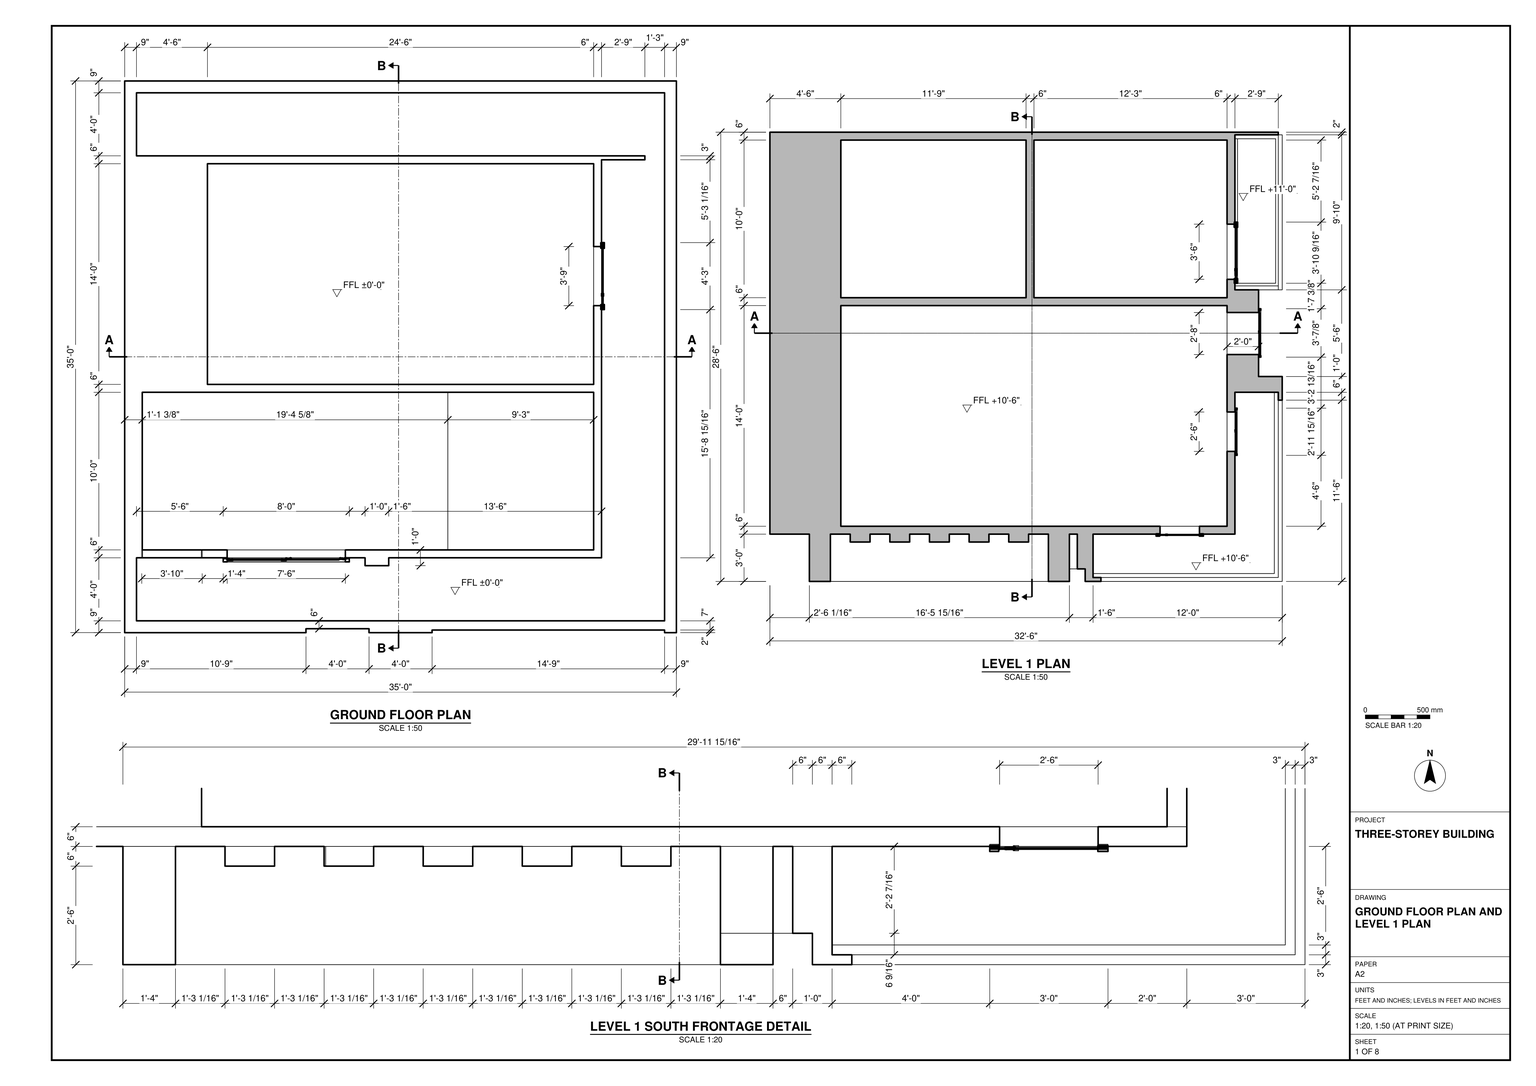
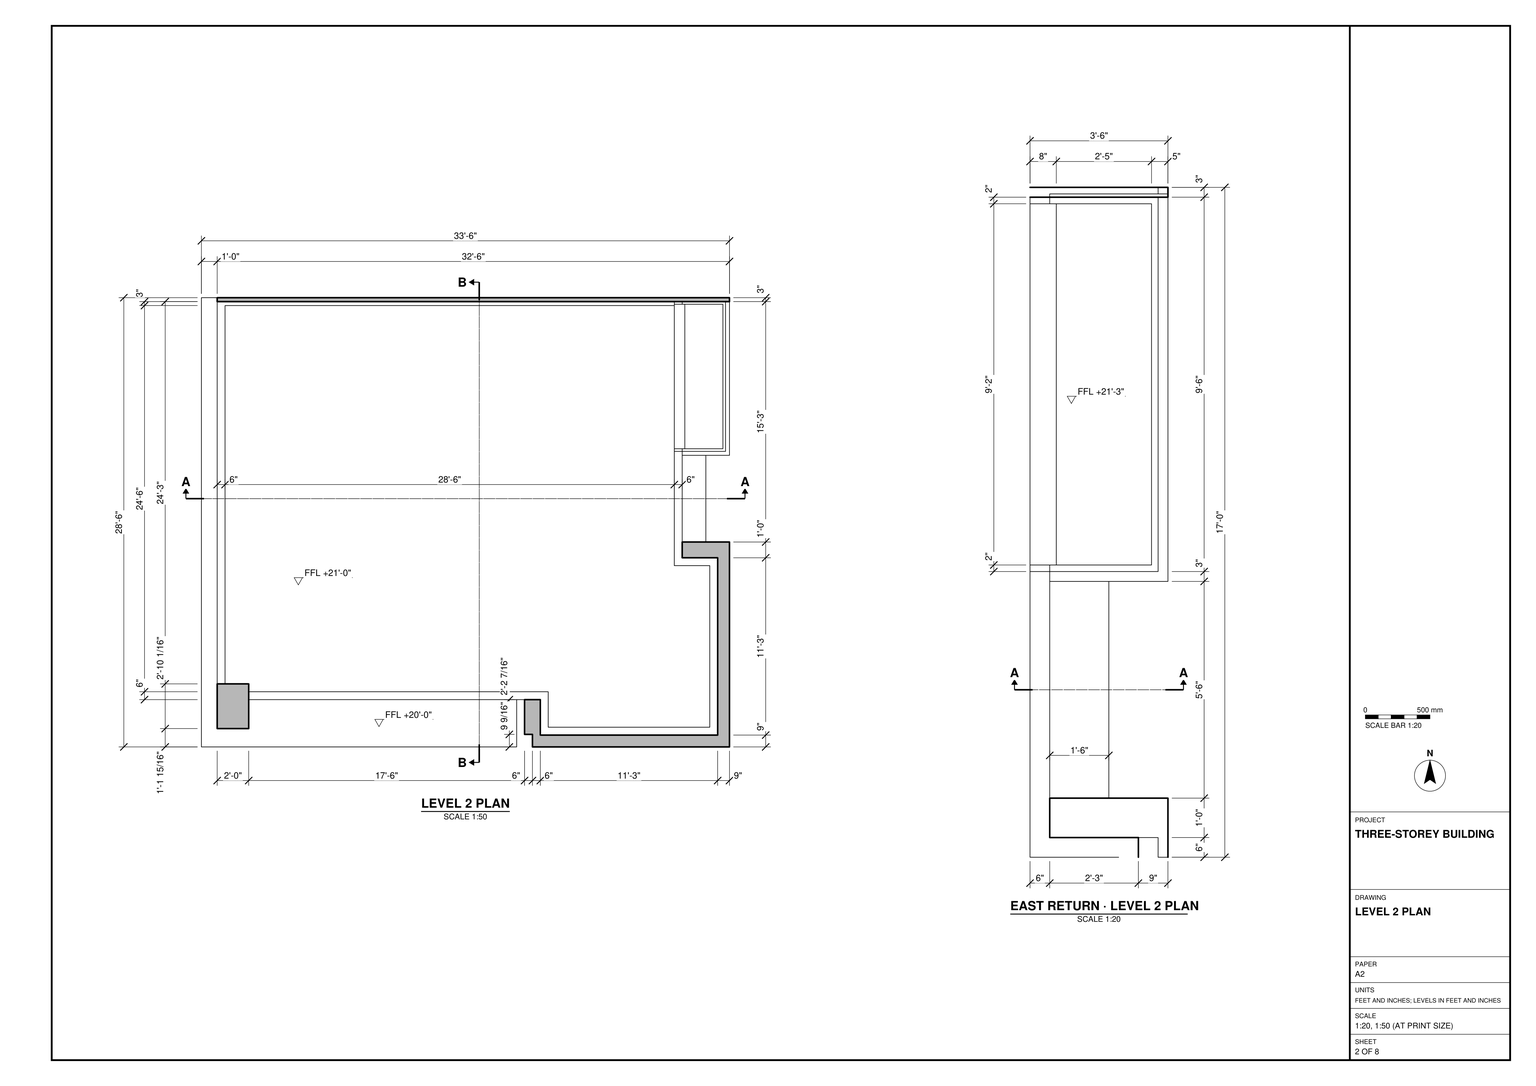
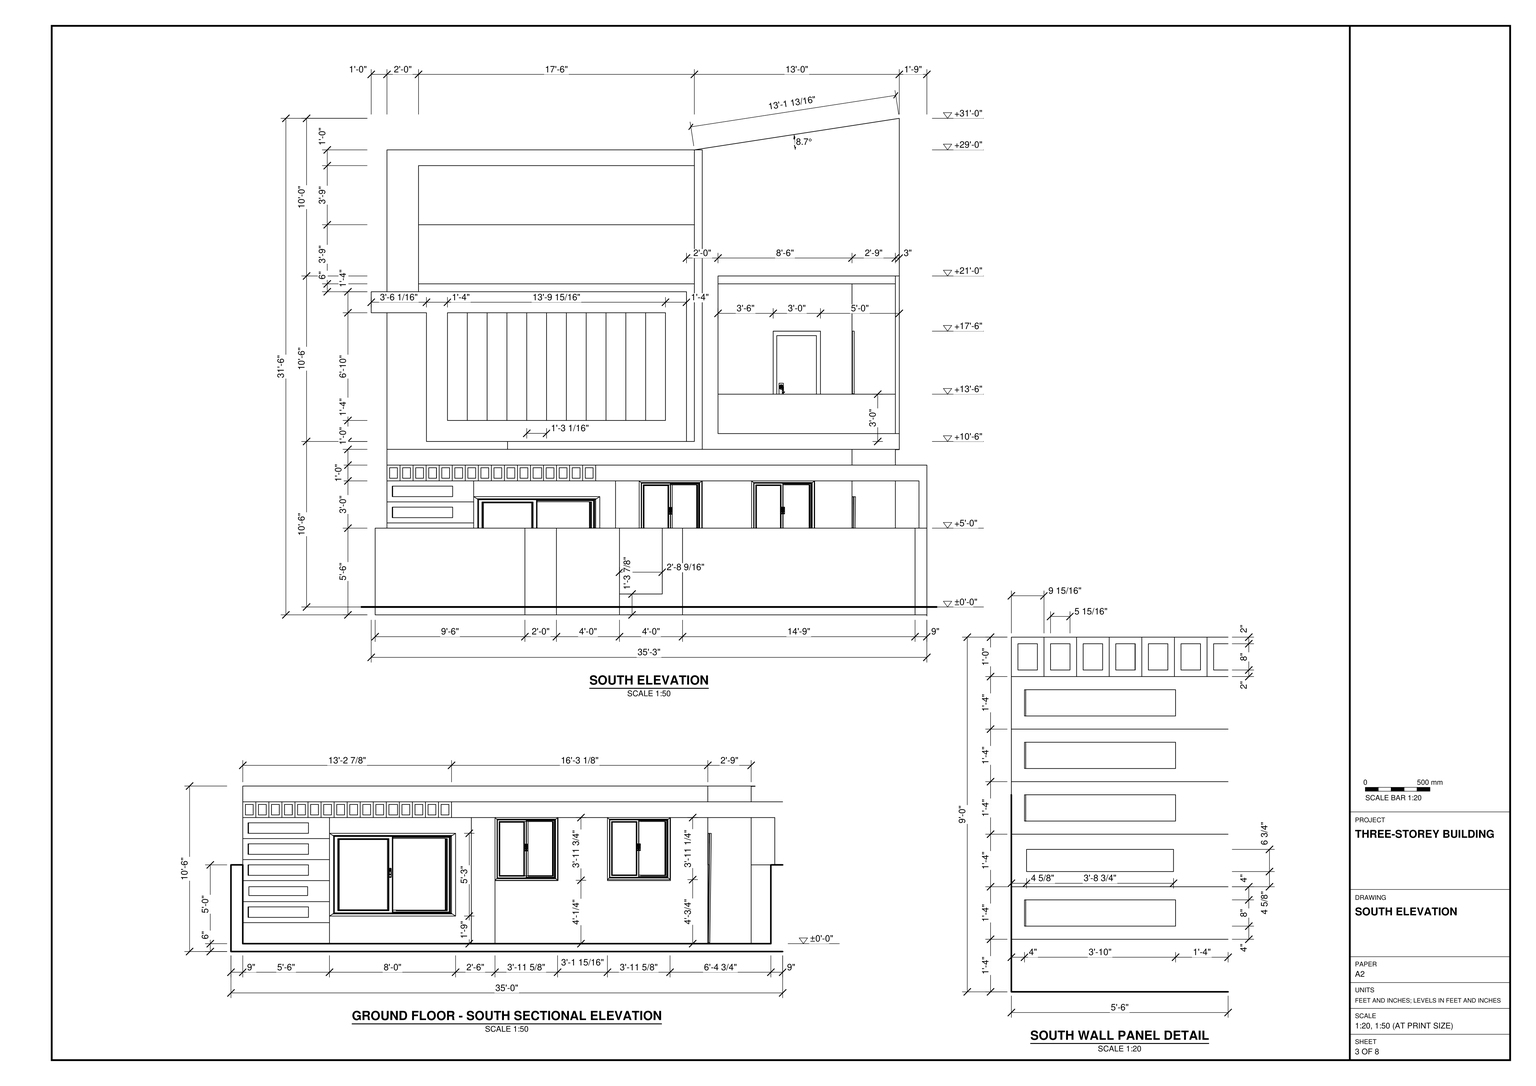
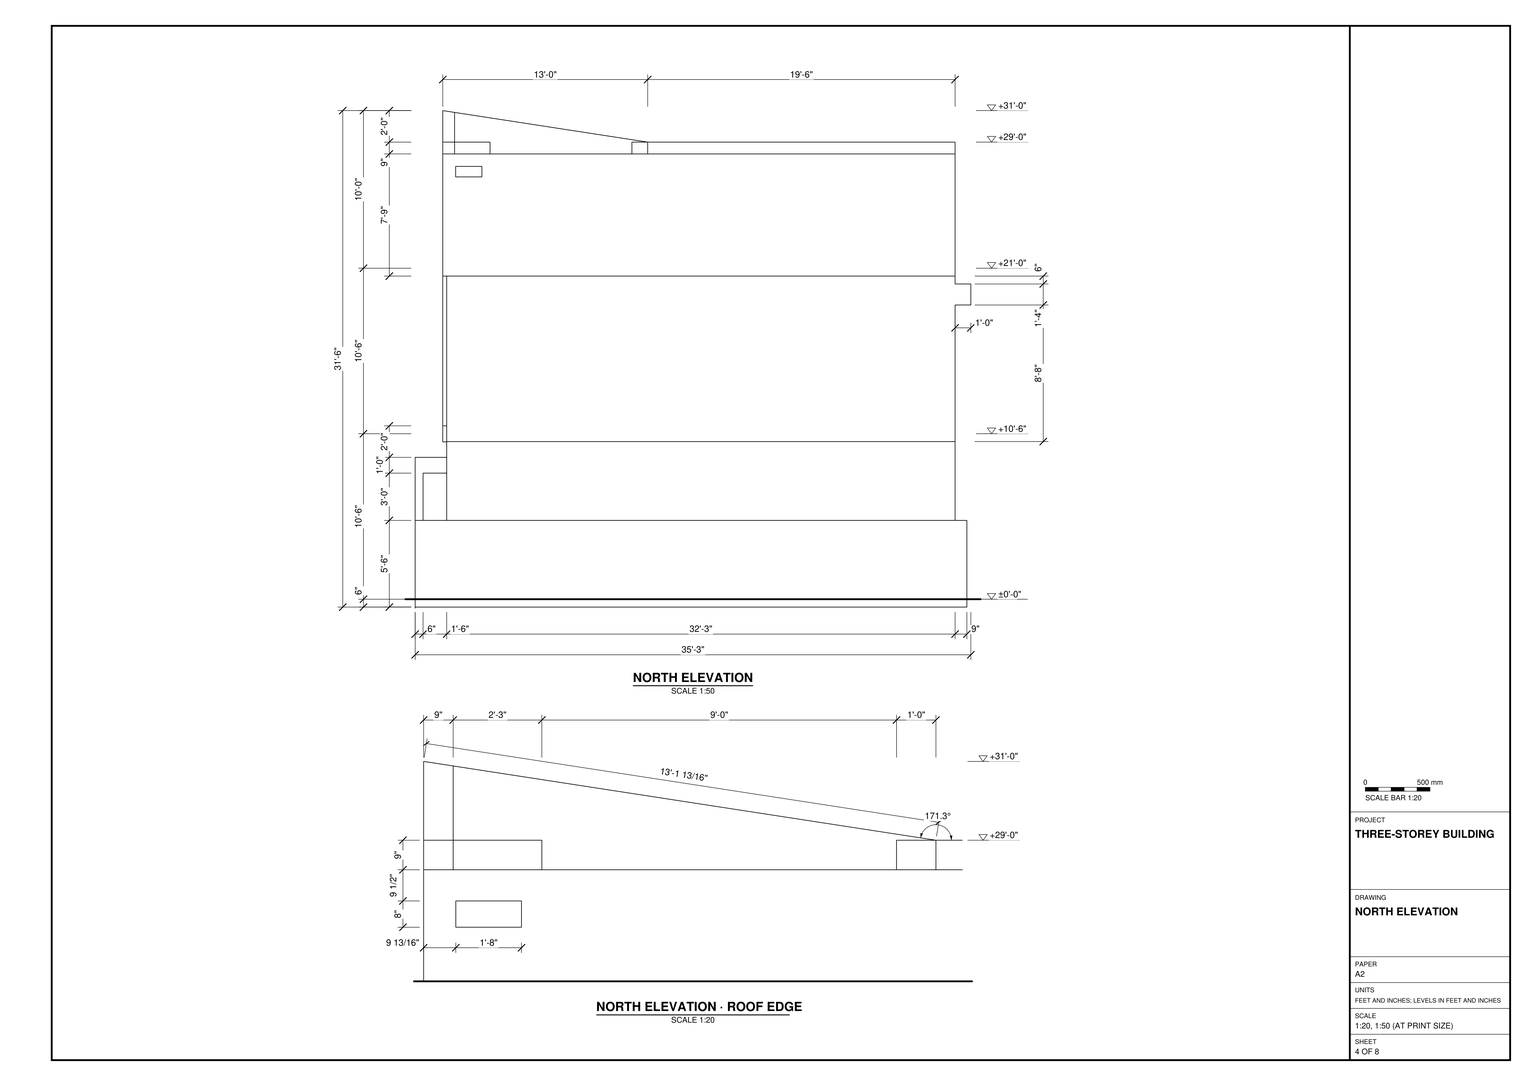
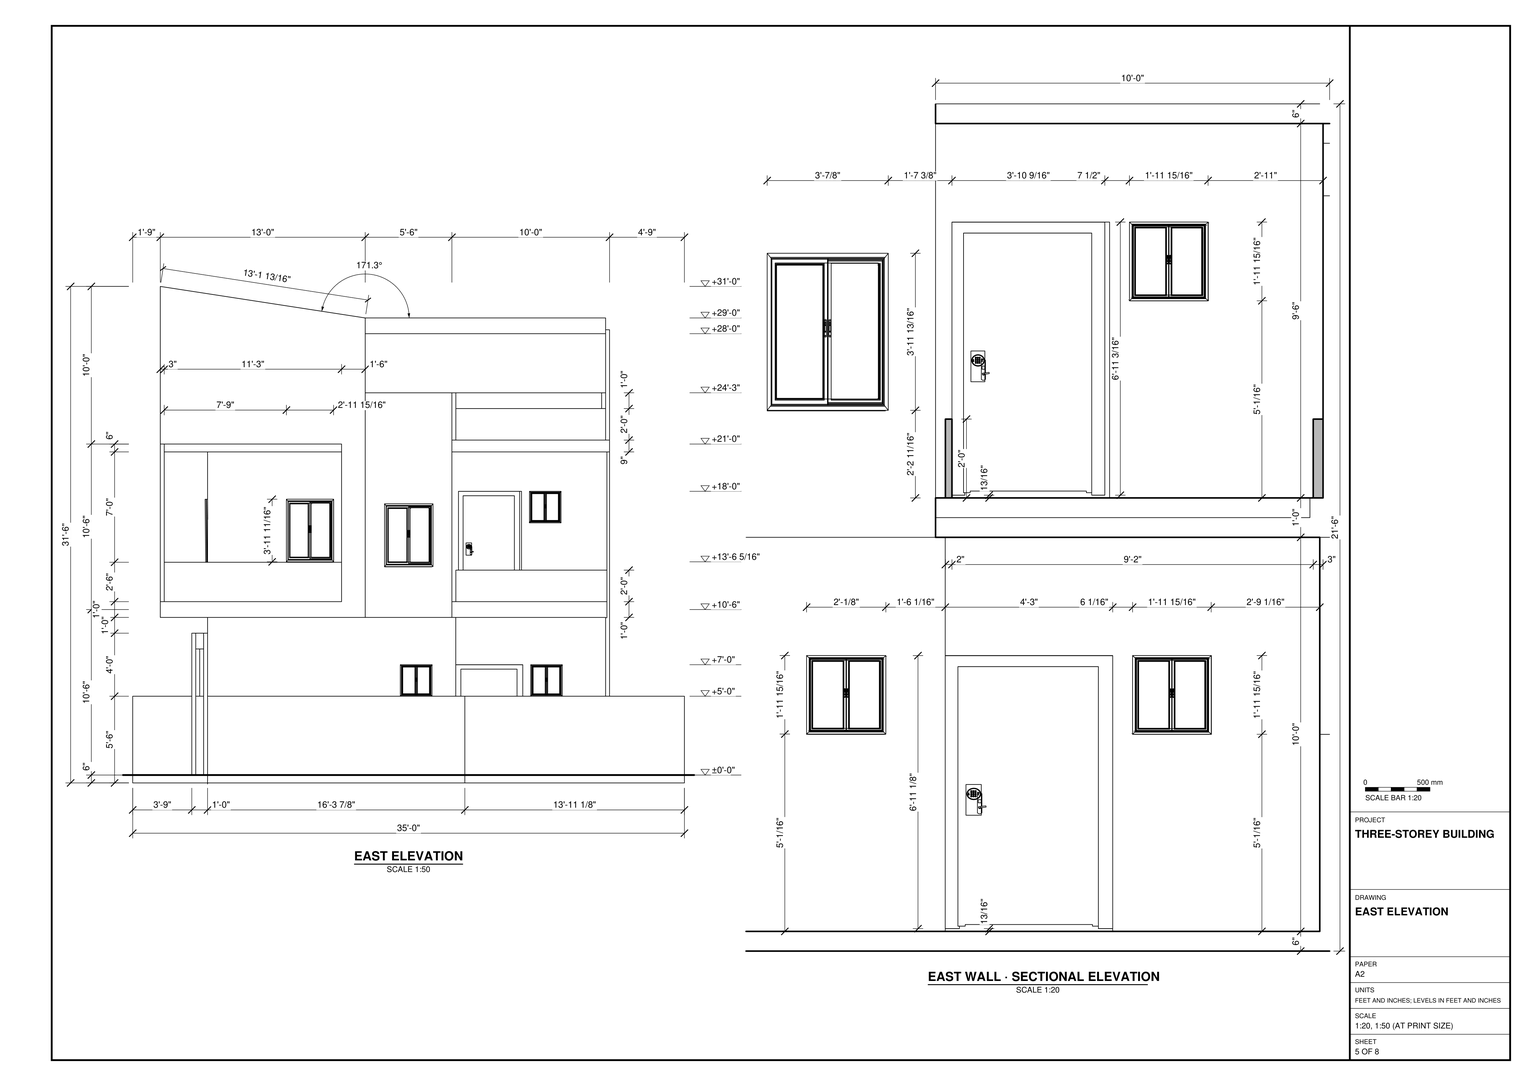
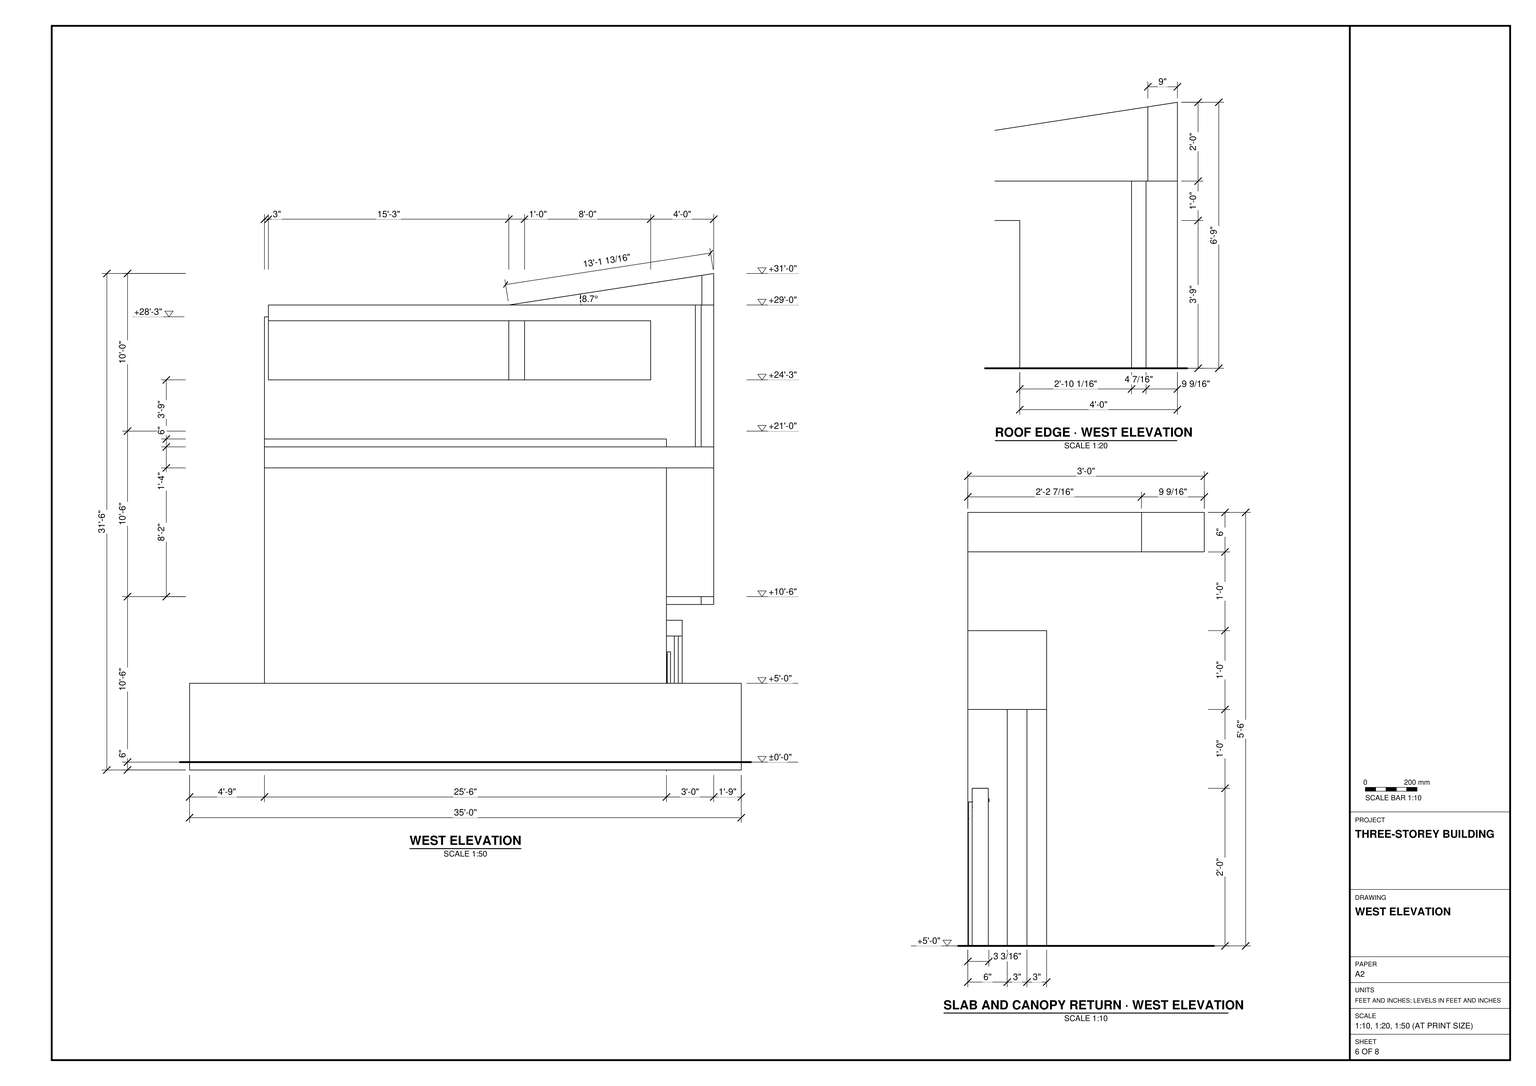
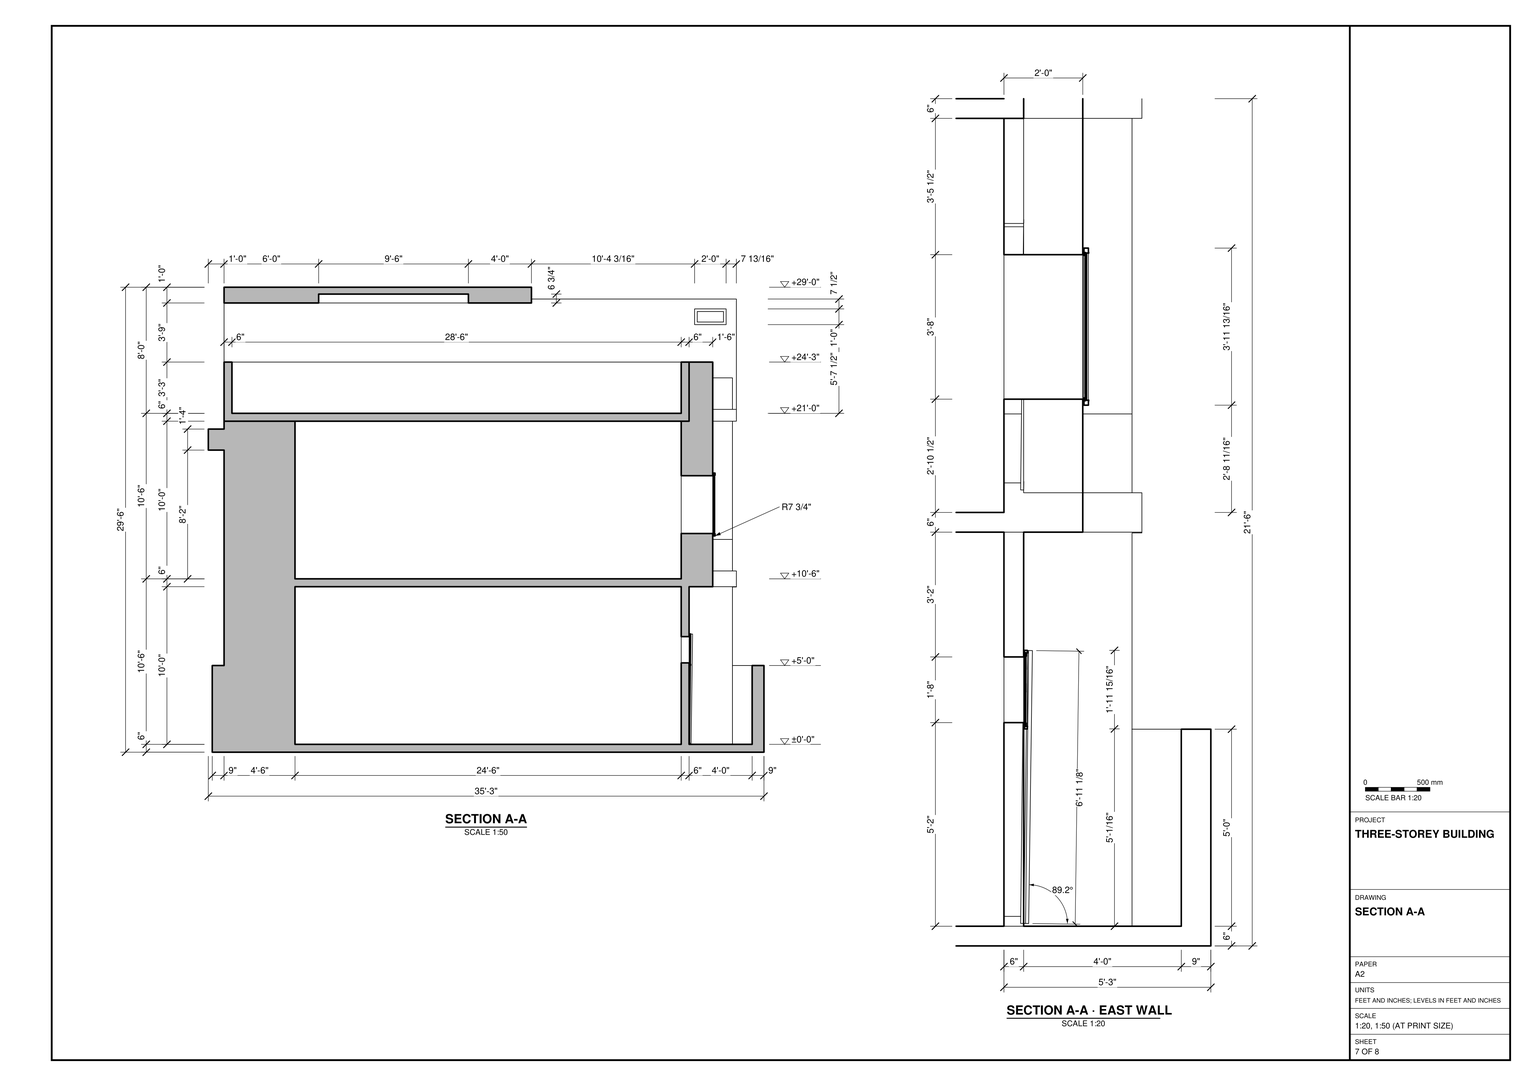
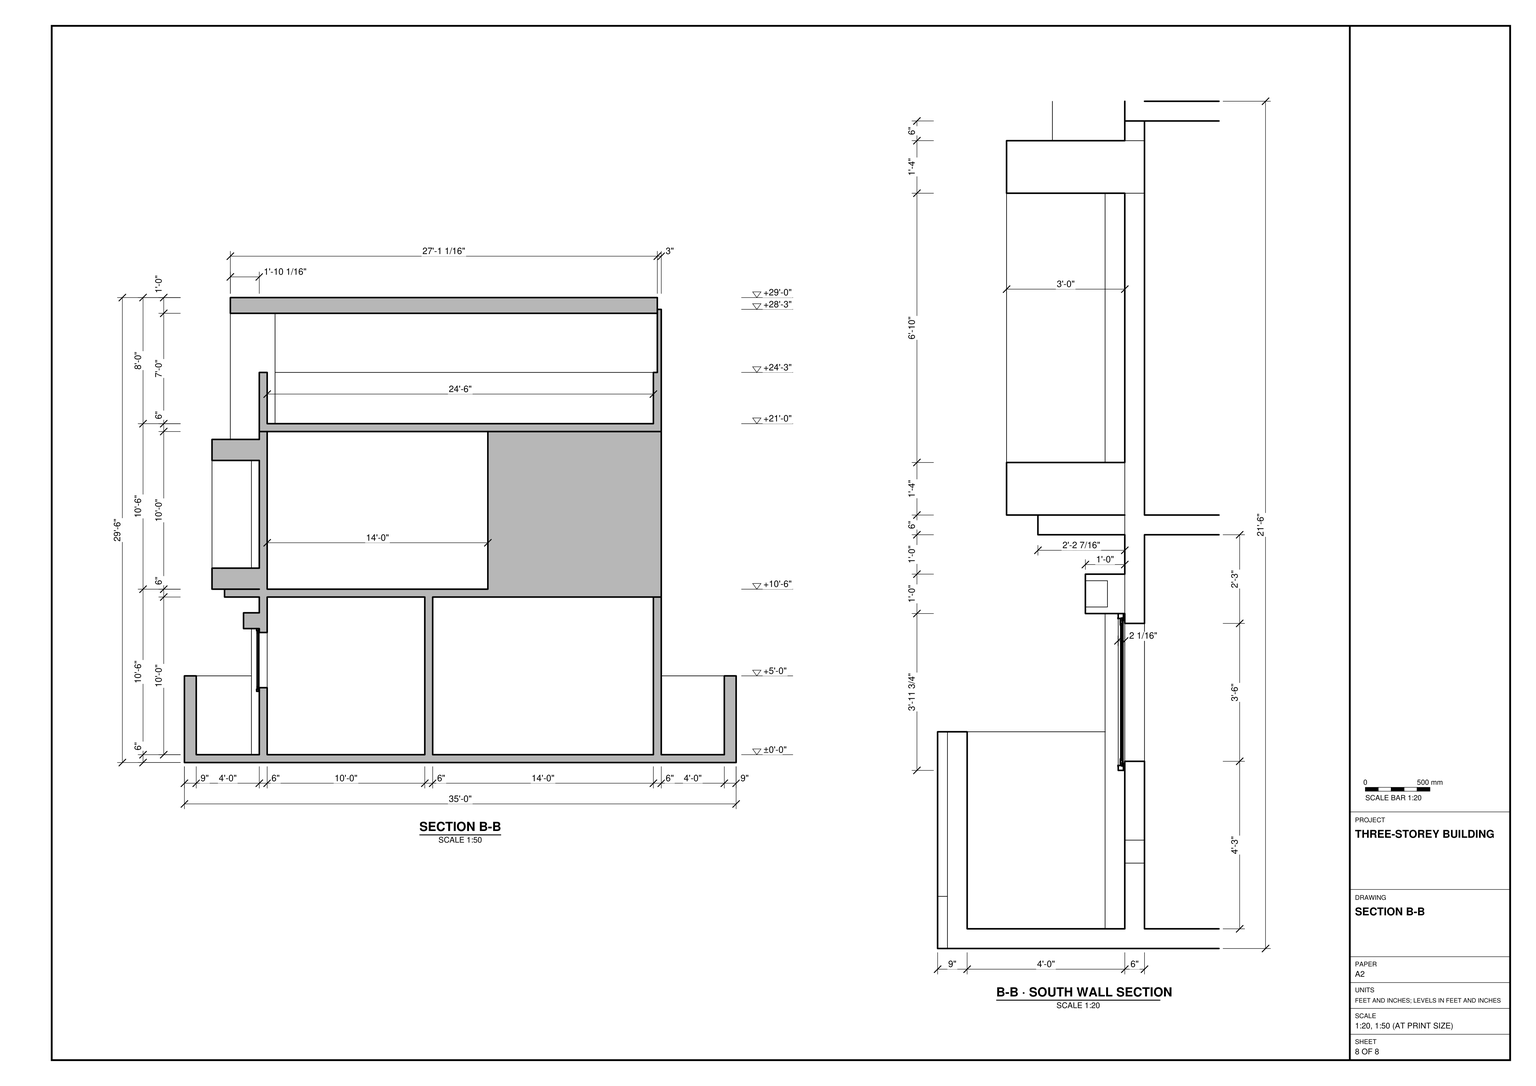
Build the three-storey building in SketchUp using task_files/diagram_01.pdf. Work in feet and inches. Orient the model with the x-axis running east–west and the y-axis running north–south. The overall extents are 35'-3" along x, 35'-0" along y and 31'-6" in height. Set the ground floor at ±0'-0", Level 1 at +10'-6" and Level 2 at +21'-0".

Use the plans to set out the perimeter wall, the space between it and the building, and the walls and slabs at each storey. Follow the wall thicknesses and slab outlines as drawn rather than repeating one footprint up the building. At ground level, use the south sectional elevation to place the framed openings and the patterned wall panel behind the perimeter wall. At Level 1, model the rear dividing wall, the projecting frame with vertical screen members on the south face, and the recessed balcony beside it. Follow the Level 2 plan for the stepped frontage and east return. Match the roof outline to the south elevation, including the change from a level edge to a rising edge over the east bay.

Keep shell elements such as walls, slabs and roof in separate groups or components. Keep each furniture or joinery piece shown separate and use components for repeated parts. Any decor or loose items shown may be represented by suitable library components. Save one SketchUp model as output_files/three_storey_building_with_a_screened_south_frontage.skp.

# SketchUp Ruby script. Lengths in inches.
U = 1.inch
M = Sketchup.active_model
def pt(a) = Geom::Point3d.new(a.map { |v| v * U })
def face(e, loops, mat)
  f = e.add_face(loops[0].map { |a| pt(a) })
  loops[1..].each { |l| e.add_face(l.map { |a| pt(a) }).erase! }
  f.material = f.back_material = mat if mat
  f
end
# faces: each face lists its corners as indices into pts; further lists are holes
def faces(e, pts, list, mat = nil) = list.each { |f| face(e, (f[0].is_a?(Array) ? f : [f]).map { |l| l.map { |i| pts[i] } }, mat) }
# xy, xz, yz: faces in a plane at the given z, y or x. An outline is a flat list of corners, or four numbers for a rectangle; further outlines are holes
def ring(l) = l.size == 4 ? [[l[0], l[1]], [l[2], l[1]], [l[2], l[3]], [l[0], l[3]]] : l.each_slice(2).to_a
def flat(e, list, mat, &to3) = list.each { |f| face(e, (f[0].is_a?(Array) ? f : [f]).map { |l| ring(l).map { |u, v| to3.(u, v) } }, mat) }
def xy(e, z, list, mat = nil) = flat(e, list, mat) { |x, y| [x, y, z] }
def xz(e, y, list, mat = nil) = flat(e, list, mat) { |x, z| [x, y, z] }
def yz(e, x, list, mat = nil) = flat(e, list, mat) { |y, z| [x, y, z] }
def lines(e, pts, list) = list.each { |a, b| e.add_line(pt(pts[a]), pt(pts[b])) }
# prism: a flat outline (further loops are holes) pulled along v
def prism(e, loops, v, mat = nil)
  f = face(e, loops, mat); d = Geom::Vector3d.new(v.map { |x| x * U })
  f.pushpull(f.normal.samedirection?(d) ? d.length : -d.length)
end
def box(e, o, s, mat = nil) = prism(e, [[o, [o[0] + s[0], o[1], o[2]], [o[0] + s[0], o[1] + s[1], o[2]], [o[0], o[1] + s[1], o[2]]]], [0, 0, s[2]], mat)
def at(x, y, z, deg = 0) = Geom::Transformation.translation(pt([x, y, z])) * Geom::Transformation.rotation(ORIGIN, Z_AXIS, deg.degrees)
def axes(o, x, y, z) = Geom::Transformation.new([*x, 0, *y, 0, *z, 0, *pt(o).to_a, 1])
def part(name) = M.definitions.add(name)
# library, detail: a bought-in or finely detailed component or shape, given as its bounding box
def library(name, o, s) = part(name).tap { |d| box(d.entities, o, s) }
def detail(e, o, s) = box(e.add_group.entities, o, s)
def put(e, d, t, mat = nil) = e.add_instance(d, t).tap { |i| i.material = mat if mat }
def group(e, t, mat = nil) = e.add_group.tap { |g| g.transformation = t; g.material = mat if mat }.entities
root = M.entities
M.materials.add("96_96_96").color = [96, 96, 96]
M.materials.add("C05_Golden_Blaze").color = [255, 123, 0]
M.materials.add("Glass_Basic_01").color = [145, 153, 153]
M.materials["Glass_Basic_01"].alpha = 0.25
M.materials.add("Glass_Basic_1").color = [161, 173, 186]
M.materials["Glass_Basic_1"].alpha = 0.25
M.materials.add("I01_Sky_Frost").color = [235, 236, 255]
M.materials.add("Metal_06_1K").color = [238, 236, 231]
M.materials.add("Plaster_04_1K").color = [100, 89, 106]
M.materials.add("Plywood_01_1K").color = [125, 96, 64]
M.materials.add("Roofing_02_1K").color = [178, 216, 135]
M.materials.add("Wood_Floor_12_1K").color = [92, 75, 65]
M.materials.add("Wood_Planks_01_1K").color = [118, 116, 119]
M.materials.add("Wood_Veneer_15_1K").color = [103, 69, 45]
M.materials.add("[Cladding_Siding_White]1").color = [207, 207, 207]
M.materials.add("[_0053_Ivory_]").color = [200, 200, 200]
c1 = library("porta+4",[0.2,-5.42,1.33],[46.55,4.72,83.21])
c2 = library("mesh-165",[-1596.32,-2661.67,-39.91],[1702.88,1739.15,82.5])
c3 = part("Group15")
put(c3.entities,c2,at(294.66,859.51,3.5))
g1 = group(root,at(3,0,0))
xy(g1,0,[[0,0,0,420,420,420,420,0,411,0,411,2,234,2,234,0,186,0,186,3,138,3,138,0]])
xy(g1,6,[[9,9,411,9,411,411,9,411,9,363,396,363,396,360,363,360,363,57,201,57,201,51,183,51,183,57,9,57],[13.377,63,246,183],[246,63,357,183],[63,189,357,357]])
xy(g1,9,[[357,248.949,363,293.949]])
xy(g1,26,[[13,57,59,63]])
xy(g1,33,[[78,57,168,63]])
xy(g1,34,[[13,57,59,63]])
xy(g1,42.625,[[13.625,57,58.375,63]])
xy(g1,49.375,[[13.625,57,58.375,63]])
xy(g1,57,[[204,57,246,63],[289.591,57,331.591,63]])
xy(g1,58,[[13,57,59,63]])
xy(g1,66,[[0,0,138,0,138,3,186,3,186,0,234,0,234,9,9,9,9,411,411,411,411,0,420,0,420,45,414,45,414,48,420,48,420,54,414,54,414,57,420,57,420,420,0,420],[234,2,411,9],[13,57,59,63]])
xy(g1,68,[[357,205.731,363,225.731],[357,305,363,325]])
xy(g1,74,[[13,57,59,63]])
xy(g1,82,[[13,57,59,63]])
xy(g1,87,[[78,57,168,63],[357,248.949,363,293.949]])
xy(g1,88,[[357,205.731,363,225.731],[357,305,363,325]])
xy(g1,90,[[13,57,59,63]])
xy(g1,98,[[13,57,59,63]])
xy(g1,99,[[204,57,246,63],[289.591,57,328.591,63],[328.591,57,331.591,63]])
xy(g1,102,[[9,45,75,57],[75,45,75,57,183,57,183,51,201,51,201,57,414,57,414,54,363,54,363,48,414,48,414,45]],"Metal_06_1K")
xy(g1,104,[[11,45,16.925,51.494],[20.931,45,26.862,51.494],[30.862,45,36.793,51.494],[40.793,45,46.649,51.494],[50.724,45,56.656,51.494],
  [60.656,45,66.587,51.721],[70.587,45,76.518,51.721],[80.518,45,86.449,51.721],[90.449,45,96.38,51.721],[100.38,45,106.311,51.721],
  [110.311,45,116.242,51.721],[120.242,45,126.787,51.721],[130.173,45,136.104,51.721],[140.104,45,146.035,51.721],[150.035,45,155.967,51.721],
  [159.967,45,165.898,51.721]],"Metal_06_1K")
xy(g1,112,[[11,45,16.925,51.494],[20.931,45,26.862,51.494],[30.862,45,36.793,51.494],[40.793,45,46.649,51.494],[50.724,45,56.656,51.494],
  [60.656,45,66.587,51.721],[70.587,45,76.518,51.721],[80.518,45,86.449,51.721],[90.449,45,96.38,51.721],[100.38,45,106.311,51.721],
  [110.311,45,116.242,51.721],[120.242,45,126.787,51.721],[130.173,45,136.104,51.721],[140.104,45,146.035,51.721],[150.035,45,155.967,51.721]])
xy(g1,112,[[159.967,45,165.898,51.721]],"Metal_06_1K")
xy(g1,114,[[9,45,243,57],[243,45,420,45,420,48,363,48,363,54,420,54,420,57,243,57]],"Metal_06_1K")
xy(g1,125.772,[[396,360,399,361]])
xy(g1,126,[[249,21,249,30.549,100.787,30.549,100.787,57,363,57,363,360,399,360,399,243,381,243,381,177,399,177,399,21],[13.377,63,357,183],[357,63,363,183],[63,189,357,357],[57,357,357,363]])
xy(g1,132,[[255,27,393,27,393,165,363,165,363,57,255,57],[100.787,30.549,237,57],[237,30.549,243,57],[63,63,357,231],[63,237,204,357],
  [210,237,357,357]])
xy(g1,132,[[39.051,21,39.051,57,100.787,57,100.787,30.549,237,30.549,237,21]],"Wood_Planks_01_1K")
xy(g1,135,[[306,57,336,63]])
xy(g1,138,[[261,21,399,21,399,159,396,159,396,24,261,24],[255,24,396,24,396,165,393,165,393,27,255,27],[363,243,396,246],[396,243,399,361],[363,246,396,246,396,361,394,361,394,248,363,248],
  [363,248,365,358],[365,248,394,358],[363,358,365,361],[365,358,394,361]])
xy(g1,141,[[357,251,363,293]])
xy(g1,148,[[55.051,21,221,21,221,57,205.914,57,205.914,51,190.827,51,190.827,57,175.741,57,175.741,51,160.655,51,160.655,57,145.569,57,145.569,51,130.482,51,130.482,57,115.396,57,115.396,51,100.31,51,100.31,57,85.223,57,85.223,51,70.137,51,70.137,57,55.051,57]],"Wood_Planks_01_1K")
xy(g1,162,[[363,246,396,246,396,361,363,361,363,358,394,358,394,248,363,248]])
xy(g1,166.5,[[357,193.731,381,225.731]])
xy(g1,168,[[255,24,396,24,396,165,393,165,393,27,255,27]])
xy(g1,171,[[357,120,363,150]])
xy(g1,200,[[357,304.051,363,324.051]])
xy(g1,210.5,[[357,193.731,381,225.731]])
xy(g1,213,[[306,57,336,63],[357,120,363,150]])
xy(g1,219,[[357,251,363,293]])
xy(g1,220,[[357,304.051,363,324.051]])
xy(g1,230,[[55.051,51,70.137,57],[85.223,51,100.31,57],[115.396,51,130.482,57],[145.569,51,160.655,57],[175.741,51,190.827,57],
  [205.914,51,221,57]],"C05_Golden_Blaze")
xy(g1,230,[[-3,21,39.051,57],[55.051,21,221,51],[-3,57,9,363]],"Wood_Planks_01_1K")
xy(g1,246,[[-3,21,237,21,237,57,33,57,33,34.962,9,34.962,9,363,-3,363]],"Wood_Planks_01_1K")
xy(g1,252,[[9,57,243,63],[243,57,357,63],[357,57,363,177],[9,63,63,231],[63,63,357,231],
  [357,177,363,231],[9,231,363,231,363,237,210,237,210,357,363,357,363,361,396,361,396,363,9,363,9,357,204,357,204,237,9,237],[9,237,63,357],[63,237,204,357],[210,237,357,357],
  [357,237,363,357],[363,243,399,357],[363,357,399,361],[396,361,399,363]])
xy(g1,252,[[255,24,255,57,363,57,363,165,396,165,396,24]],"I01_Sky_Frost")
xy(g1,258,[[261,21,261,24,396,24,396,159,399,159,399,21],[261,36,384,36,384,159,357,159,357,357,15,357,15,69,33,69,33,63,261,63]])
xy(g1,261,[[363,243,399,243,399,360,396,360,396,246,363,246],[357,246,363,248],[363,246,396,246,396,360,363,360,363,358,394,358,394,248,363,248],[357,248,365,358],[365,248,394,358],
  [357,358,363,360]])
xy(g1,285,[[363,246,396,246,396,360,363,360,363,358,394,358,394,248,363,248]])
xy(g1,297,[[255,30,390,30,390,165,363,165,363,246,357,246,357,159,384,159,384,36,261,36,261,63,33,63,33,57,255,57],[9,69,15,69,15,357,357,357,357,360,9,360],[363,177,381,243]])
xy(g1,327.507,[[369.196,360,389.196,363]],"Wood_Veneer_15_1K")
xy(g1,335.507,[[369.196,360,389.196,363]],"Wood_Veneer_15_1K")
xy(g1,342,[[[33,34.962,243,360],[81,82.962,195,312]],[9,69,33,360]])
xy(g1,345,[[9,360,399,363]])
xy(g1,348.766,[[81,82.962,195,312]],"Wood_Floor_12_1K")
xy(g1,354,[[243,30,249,30.549],[249,30,255,30,255,57,243,57,243,30.549,249,30.549],[9,34.962,243,360],[363,165,390,177]])
xy(g1,354,[[243,21,249,30]],"Wood_Planks_01_1K")
xz(g1,0,[[114,0,138,66],[186,0,234,0,234,66,218.552,66,218.552,15.871,186,15.871],[411,0,420,66]])
xz(g1,0,[[0,0,114,66]],"Plywood_01_1K")
xz(g1,0,[[186,15.871,218.552,66]],"Roofing_02_1K")
xz(g1,2,[[234,0,411,66]],"Plywood_01_1K")
xz(g1,3,[[138,0,186,66]],"Plaster_04_1K")
xz(g1,9,[[9,6,411,66]])
xz(g1,21,[[249,126,399,126,399,138,261,138,261,258,399,258,399,378,243,354,249,354],[[39.051,132,237,132,237,246,-3,246,-3,230,39.051,230],[55.051,148,221,230]]],"Wood_Planks_01_1K")
xz(g1,24,[[255,138,261,168],[255,168,261,252]])
xz(g1,24,[[261,138,396,168]],"Glass_Basic_01")
xz(g1,24,[[261,252,396,258]],"I01_Sky_Frost")
xz(g1,27,[[255,132,393,138]])
xz(g1,27,[[255,138,393,168]],"Glass_Basic_01")
xz(g1,30,[[255,297,255,354,243,354,390,376.615,390,297]])
xz(g1,30.549,[[100.787,126,249,126,249,354,243,354,243,132,100.787,132]])
xz(g1,34.962,[[9,246,33,246,33,342,243,342,243,354,9,354]],"I01_Sky_Frost")
xz(g1,36,[[261,258,384,297]])
xz(g1,45,[[16.925,104,16.931,112],[46.649,104,46.724,112]])
xz(g1,45,[[414,66,420,66,420,114,167.898,114,167.898,102,414,102],[[9,102,18.931,114],[11,104,16.931,112]],[[18.931,102,28.862,114],[20.931,104,26.862,112]],[[28.862,102,38.793,114],[30.862,104,36.793,112]],[[38.793,102,48.724,114],[40.793,104,46.724,112]],
  [[48.724,102,58.656,114],[50.724,104,56.656,112]],[[58.656,102,68.587,114],[60.656,104,66.587,112]],[[68.587,102,78.518,114],[70.587,104,76.518,112]],[[78.518,102,88.449,114],[80.518,104,86.449,112]],[[88.449,102,98.38,114],[90.449,104,96.38,112]],
  [[98.38,102,108.311,114],[100.38,104,106.311,112]],[[108.311,102,118.242,114],[110.311,104,116.242,112]],[[118.242,102,128.173,114],[120.242,104,126.787,112]],[[128.173,102,138.104,114],[130.173,104,136.104,112]],[[138.104,102,148.035,114],[140.104,104,146.035,112]],
  [[148.035,102,157.967,114],[150.035,104,155.967,112]],[[157.967,102,167.898,114],[159.967,104,165.898,112]]],"Metal_06_1K")
xz(g1,48,[[414,66,414,102,363,102,363,114,420,114,420,66]],"Metal_06_1K")
xz(g1,51,[[70.137,148,85.223,230],[100.31,148,115.396,230],[130.482,148,145.569,230],[160.655,148,175.741,230],[190.827,148,205.914,230]])
xz(g1,51,[[183,6,201,102]],"[_0053_Ivory_]")
xz(g1,51.494,[[11,104,16.925,112],[20.931,104,26.862,112],[30.862,104,36.793,112],[40.793,104,46.649,112],[50.724,104,56.656,112]],"Metal_06_1K")
xz(g1,51.721,[[60.656,104,66.587,112],[70.587,104,76.518,112],[80.518,104,86.449,112],[90.449,104,96.38,112],[100.38,104,106.311,112],
  [110.311,104,116.242,112],[120.242,104,126.787,112],[130.173,104,136.104,112],[140.104,104,146.035,112],[150.035,104,155.967,112],
  [159.967,104,165.898,112]],"Metal_06_1K")
xz(g1,54,[[414,66,420,66,420,114,363,114,363,102,414,102]],"Metal_06_1K")
xz(g1,57,[[9,6,75,22],[201,6,363,6,363,102,334.591,102,334.591,54,286.591,54,286.591,102,249,102,249,54,201,54],[[75,30,171,90],[78,33,168,87]],[[201,54,249,102],[204,57,246,99]],[[286.591,54,334.591,102],[289.591,57,331.591,99]],
  [9,114,363,126],[9,126,100.787,126,100.787,132,39.051,132,39.051,230,9,230],[237,132,243,132,243,252,33,252,33,246,237,246],[[303,132,339,216],[306,135,336,213]],[55.051,148,70.137,230],
  [85.223,148,100.31,230],[115.396,148,130.482,230],[145.569,148,160.655,230],[175.741,148,190.827,230],[205.914,148,221,230],
  [9,246,33,252],[243,252,255,297],[243,297,255,354]])
xz(g1,57,[[[9,22,75,38],[13,26,59,34]],[[9,38,75,54],[13.625,42.625,58.375,49.375]],[[9,54,75,70],[13,58,59,66]],[[9,70,75,86],[13,74,59,82]],[[9,86,75,102],[13,90,59,98]]],"96_96_96")
xz(g1,57,[[255,132,303,132,303,216,339,216,339,132,363,132,363,252,255,252],[33,252,243,297]],"I01_Sky_Frost")
xz(g1,57,[[414,66,414,102,363,102,363,114,420,114,420,66]],"Metal_06_1K")
xz(g1,57,[[75,6,183,6,183,102,75,102,75,90,171,90,171,30,75,30]],"[_0053_Ivory_]")
xz(g1,63,[[[13.377,6,13.377,26,59,26,59,34,13.377,34,13.377,58,59,58,59,66,13.377,66,13.377,74,59,74,59,82,13.377,82,13.377,90,59,90,59,98,13.377,98,13.377,126,246,126,246,99,204,99,204,57,246,57,246,6],[78,33,168,87],[13.625,42.625,58.375,49.375]],[[246,6,357,126],[289.591,57,331.591,99]],[13,26,13.377,34],[13,58,13.377,66],[13,74,13.377,82],
  [13,90,13.377,98],[63,132,243,252],[[243,132,357,252],[306,135,336,213]],[33,258,243,297],[243,258,261,297]])
xz(g1,69,[[15,258,33,297],[9,297,33,342]])
xz(g1,82.962,[[81,342,195,348.766]])
xz(g1,120,[[357,171,363,213]])
xz(g1,150,[[357,171,363,213]])
xz(g1,159,[[396,138,399,258],[357,258,384,297]])
xz(g1,165,[[393,138,396,168],[363,297,390,354]])
xz(g1,165,[[363,132,393,132,393,168,396,168,396,252,363,252]],"Wood_Veneer_15_1K")
xz(g1,177,[[381,126,390,132],[381,132,381,297,363,297,363,354,390,354,390,132]])
xz(g1,177,[[390,126,399,132],[390,132,399,354]],"Wood_Planks_01_1K")
xz(g1,183,[[13.377,6,357,126]])
xz(g1,189,[[63,6,357,126]])
xz(g1,193.731,[[357,166.5,381,210.5]])
xz(g1,205.731,[[357,68,363,88]])
xz(g1,225.731,[[357,68,363,88],[357,166.5,381,210.5]])
xz(g1,231,[[63,132,357,252]])
xz(g1,237,[[63,132,204,252],[210,132,357,252]])
xz(g1,243,[[363,138,381,252],[363,252,381,261],[363,261,381,297]])
xz(g1,243,[[381,126,399,138],[381,252,399,261]],"I01_Sky_Frost")
xz(g1,246,[[357,261,363,297]])
xz(g1,246,[[363,138,396,162],[363,261,396,285]],"Glass_Basic_1")
xz(g1,248,[[363,138,394,162],[363,261,394,285]],"Glass_Basic_1")
xz(g1,248.949,[[357,9,363,87]])
xz(g1,251,[[357,141,363,162],[357,162,363,219]])
xz(g1,293,[[357,141,363,219]])
xz(g1,293.949,[[357,9,363,87]])
xz(g1,304.051,[[357,200,363,220]])
xz(g1,305,[[357,68,363,88]])
xz(g1,312,[[81,342,195,348.766]])
xz(g1,324.051,[[357,200,363,220]])
xz(g1,325,[[357,68,363,88]])
xz(g1,357,[[63,6,357,126],[63,132,204,252],[210,132,357,252],[15,258,357,297]])
xz(g1,358,[[363,138,394,162],[363,261,394,285]],"Glass_Basic_1")
xz(g1,360,[[363,261,396,285],[[367.196,325.507,391.196,337.507],[369.196,327.507,389.196,335.507]],[9,345,243,354]])
xz(g1,360,[[363,261,396,285]],"Glass_Basic_1")
xz(g1,360,[[363,6,396,6,396,125.772,399,125.772,399,126,363,126],[[357,261,363,261,363,285,396,285,396,261,399,261,399,345,243,345,243,342,9,342,9,297,357,297],[367.196,325.507,391.196,337.507]],[9,342,243,345]],"Wood_Veneer_15_1K")
xz(g1,361,[[396,125.772,399,138],[363,138,396,162]])
xz(g1,361,[[363,162,396,252]],"Wood_Veneer_15_1K")
xz(g1,363,[[9,6,396,126],[9,126,9,230,-3,230,-3,246,9,246,9,252,396,252,396,126],[[9,252,399,345],[369.196,327.507,389.196,335.507]]])
xz(g1,411,[[9,6,411,66]])
xz(g1,420,[[0,0,420,66]])
yz(g1,-3,[[21,230,363,246]],"Wood_Planks_01_1K")
yz(g1,0,[[0,0,420,66]])
yz(g1,9,[[9,6,57,66],[363,6,411,66],[57,66,363,230],[34.962,246,34.962,354,360,354,360,342,69,342,69,297,360,297,360,345,363,345,363,252,57,252,57,246],[57,246,363,252]])
yz(g1,9,[[45,102,57,114]],"Metal_06_1K")
yz(g1,11,[[45,104,51.494,112]],"Metal_06_1K")
yz(g1,13,[[57,26,63,34],[57,58,63,66],[57,74,63,82],[57,90,63,98]])
yz(g1,13.377,[[63,6,183,126]])
yz(g1,13.625,[[57,42.625,63,49.375]])
yz(g1,15,[[69,258,357,297]])
yz(g1,16.925,[[45,104,51.494,112]],"Metal_06_1K")
yz(g1,20.931,[[45,104,51.494,112]],"Metal_06_1K")
yz(g1,26.862,[[45,104,51.494,112]],"Metal_06_1K")
yz(g1,30.862,[[45,104,51.494,112]],"Metal_06_1K")
yz(g1,33,[[34.962,246,57,246,57,297,63,297,63,258,69,258,69,342,34.962,342]],"I01_Sky_Frost")
yz(g1,36.793,[[45,104,51.494,112]],"Metal_06_1K")
yz(g1,39.051,[[21,132,57,230]],"Wood_Planks_01_1K")
yz(g1,40.793,[[45,104,51.494,112]],"Metal_06_1K")
yz(g1,46.649,[[45,104,51.494,112]],"Metal_06_1K")
yz(g1,50.724,[[45,104,51.494,112]],"Metal_06_1K")
yz(g1,55.051,[[51,148,57,230]],"C05_Golden_Blaze")
yz(g1,55.051,[[21,148,51,230]],"Wood_Planks_01_1K")
yz(g1,56.656,[[45,104,51.494,112]],"Metal_06_1K")
yz(g1,58.375,[[57,42.625,63,49.375]])
yz(g1,59,[[57,26,63,34],[57,58,63,66],[57,74,63,82],[57,90,63,98]])
yz(g1,60.656,[[45,104,51.721,112]],"Metal_06_1K")
yz(g1,63,[[189,6,357,126],[63,132,231,252],[237,132,357,252]])
yz(g1,66.587,[[45,104,51.721,112]],"Metal_06_1K")
yz(g1,70.137,[[51,148,57,230]])
yz(g1,70.587,[[45,104,51.721,112]],"Metal_06_1K")
yz(g1,76.518,[[45,104,51.721,112]],"Metal_06_1K")
yz(g1,78,[[57,33,63,87]])
yz(g1,80.518,[[45,104,51.721,112]],"Metal_06_1K")
yz(g1,81,[[82.962,342,312,348.766]])
yz(g1,85.223,[[51,148,57,230]])
yz(g1,86.449,[[45,104,51.721,112]],"Metal_06_1K")
yz(g1,90.449,[[45,104,51.721,112]],"Metal_06_1K")
yz(g1,96.38,[[45,104,51.721,112]],"Metal_06_1K")
yz(g1,100.31,[[51,148,57,230]])
yz(g1,100.38,[[45,104,51.721,112]],"Metal_06_1K")
yz(g1,100.787,[[30.549,126,57,132]])
yz(g1,106.311,[[45,104,51.721,112]],"Metal_06_1K")
yz(g1,110.311,[[45,104,51.721,112]],"Metal_06_1K")
yz(g1,115.396,[[51,148,57,230]])
yz(g1,116.242,[[45,104,51.721,112]],"Metal_06_1K")
yz(g1,120.242,[[45,104,51.721,112]],"Metal_06_1K")
yz(g1,126.787,[[45,104,51.721,112]],"Metal_06_1K")
yz(g1,130.173,[[45,104,51.721,112]],"Metal_06_1K")
yz(g1,130.482,[[51,148,57,230]])
yz(g1,136.104,[[45,104,51.721,112]],"Metal_06_1K")
yz(g1,138,[[0,0,3,66]])
yz(g1,140.104,[[45,104,51.721,112]],"Metal_06_1K")
yz(g1,145.569,[[51,148,57,230]])
yz(g1,146.035,[[45,104,51.721,112]],"Metal_06_1K")
yz(g1,150.035,[[45,104,51.721,112]],"Metal_06_1K")
yz(g1,155.967,[[45,104,51.721,112]],"Metal_06_1K")
yz(g1,159.967,[[45,104,51.721,112]],"Metal_06_1K")
yz(g1,160.655,[[51,148,57,230]])
yz(g1,165.898,[[45,104,51.721,112]],"Metal_06_1K")
yz(g1,168,[[57,33,63,87]])
yz(g1,175.741,[[51,148,57,230]])
yz(g1,183,[[51,6,57,102]],"[_0053_Ivory_]")
yz(g1,186,[[0,0,3,15.871],[0,15.871,3,66]])
yz(g1,190.827,[[51,148,57,230]])
yz(g1,195,[[82.962,342,312,348.766]])
yz(g1,201,[[51,6,57,102]],"[_0053_Ivory_]")
yz(g1,204,[[57,57,63,99],[237,132,357,252]])
yz(g1,205.914,[[51,148,57,230]])
yz(g1,210,[[237,132,357,252]])
yz(g1,221,[[21,148,57,230]],"Wood_Planks_01_1K")
yz(g1,234,[[0,0,2,66]])
yz(g1,237,[[21,132,57,246]],"Wood_Planks_01_1K")
yz(g1,243,[[30.549,132,30.549,354,34.962,354,34.962,342,57,342,57,132],[34.962,342,57,354],[57,342,360,354]])
yz(g1,246,[[57,57,63,99]])
yz(g1,249,[[21,126,30.549,354]])
yz(g1,255,[[24,138,27,168],[30,297,57,354]])
yz(g1,255,[[27,132,57,132,57,252,24,252,24,168,27,168]],"Wood_Veneer_15_1K")
yz(g1,261,[[21,138,24,258],[36,258,63,297]])
yz(g1,289.591,[[57,57,63,99]])
yz(g1,306,[[57,135,63,213]])
yz(g1,331.591,[[57,57,63,99]])
yz(g1,336,[[57,135,63,213]])
yz(g1,357,[[63,6,183,126],[[189,6,357,126],[248.949,9,293.949,87],[305,68,325,88],[205.731,68,225.731,88]],[[63,132,177,252],[120,171,150,213]],[[177,132,231,252],[193.731,166.5,225.731,210.5]],[[237,132,357,252],[251,141,293,219],[304.051,200,324.051,220]],
  [159,258,177,297],[177,258,246,297],[246,258,357,261],[357,258,360,261],[357,261,360,297]])
yz(g1,363,[[[245.949,6,296.949,90],[248.949,9,293.949,87]],[[296.949,6,360,6,360,126,245.949,126,245.949,90,296.949,90],[303,66,327,90]],[[203.731,66,227.731,90],[205.731,68,225.731,88]],[[303,66,327,90],[305,68,325,88]],[48,102,54,114],
  [[243,138,246,138,246,162,248,162,248,222,296,222,296,138,358,138,358,162,361,162,361,252,243,252],[302.051,198,326.051,222]],[246,138,248,162],[[248,138,296,222],[251,141,293,219]],[358,138,361,162],[[117,168,153,216],[120,171,150,213]],
  [[302.051,198,326.051,222],[304.051,200,324.051,220]],[165,252,177,297],[177,252,231,297],[231,252,237,297],[237,252,243,297],
  [243,261,246,297],[246,261,248,285],[358,261,360,285],[165,297,177,354]])
yz(g1,363,[[[57,132,165,252],[117,168,153,216]]],"I01_Sky_Frost")
yz(g1,363,[[[57,6,245.949,126],[203.731,66,227.731,90]]],"[Cladding_Siding_White]1")
yz(g1,369.196,[[360,327.507,363,335.507]],"Wood_Veneer_15_1K")
yz(g1,381,[[[191.731,164.5,227.731,212.5],[193.731,166.5,225.731,210.5]]])
yz(g1,381,[[[177,126,243,297],[191.731,164.5,227.731,212.5]]],"[Cladding_Siding_White]1")
yz(g1,384,[[36,258,159,297]])
yz(g1,389.196,[[360,327.507,363,335.507]],"Wood_Veneer_15_1K")
yz(g1,390,[[30,297,30,376.615,177,354,165,354,165,297]])
yz(g1,393,[[27,132,165,138]])
yz(g1,393,[[27,138,165,168]],"Glass_Basic_01")
yz(g1,394,[[248,138,358,162],[248,261,358,285]],"Glass_Basic_1")
yz(g1,396,[[159,138,165,168],[159,168,165,252]])
yz(g1,396,[[24,138,159,168]],"Glass_Basic_01")
yz(g1,396,[[246,138,361,162],[246,261,360,285]],"Glass_Basic_1")
yz(g1,396,[[24,252,159,258]],"I01_Sky_Frost")
yz(g1,396,[[360,6,363,6,363,252,361,252,361,125.772,360,125.772]],"Wood_Veneer_15_1K")
yz(g1,399,[[360,125.772,361,125.772,361,138,243,138,243,126,360,126],[243,252,363,261]],"I01_Sky_Frost")
yz(g1,399,[[21,126,177,126,177,354,21,378,21,258,159,258,159,138,21,138]],"Wood_Planks_01_1K")
yz(g1,399,[[360,261,363,345]],"Wood_Veneer_15_1K")
yz(g1,411,[[0,0,2,66],[9,6,411,66]])
yz(g1,414,[[45,66,48,102],[54,66,57,102]])
yz(g1,420,[[0,0,57,0,57,6,54,6,54,66,48,66,48,6,45,6,45,66,0,66],[252.852,0,420,66]])
yz(g1,420,[[45,6,48,114],[54,6,57,114]],"Metal_06_1K")
yz(g1,420,[[57,0,252.852,66]],"Plaster_04_1K")
p = [[243,21,354],[399,21,378],[390,30,376.615],[243,30,354],[390,177,354],[399,177,354],
  [357,189,126],[363,189,126],[63,189,126],[57,189,126],[63,237,132],[63,231,132],
  [210,357,132],[204,357,132],[255,24,252],[255,24,354],[261,24,258],[261,24,354],
  [396,159,258],[396,159,354],[390,165,354],[399,165,354],[399,159,354],[390,30,354],
  [390,21,354],[261,30,354],[255,30,354],[261,21,354],[420,57,0],[420,57,-0.857]]
faces(g1,p,[[0,1,2,3],[4,2,1,5]],"Wood_Planks_01_1K")
lines(g1,p,[[6,7],[8,9],[10,11],[12,13],[14,15],[16,17],[18,19],[20,21],[19,22],[23,24],[25,17],[26,15],
  [17,27],[28,29]])
put(g1,c1,axes([302.84,58.96,130.65],[0.77339,0,0],[0,0.71,0],[0,0,1.0096]))
put(g1,c1,at(360.24,247.8,137.48,90))
put(g1,c1,axes([360.24,245.73,5.48],[0,1.09563,0],[-1,0,0],[0,0,0.99975]))
put(g1,c3,axes([323.01,56.01,103.71],[0.02798,0,0],[0,0,0.02717],[0,-0.02717,0]))
put(g1,c3,axes([237.41,56.08,103.73],[0.02797,0,0],[0,0,0.02746],[0,-0.0252,0]))
put(g1,c3,axes([148.38,55.57,92.28],[0.05638,0,0],[0,0,0.03622],[0,-0.03937,0]))
put(g1,c3,axes([381.79,219.92,214.23],[0,0.02165,0],[0,0,0.0275],[0.02165,0,0]))
put(g1,c3,axes([363.77,144.46,217.73],[0,0.02109,0],[0,0,0.02742],[0.02109,0,0]))
put(g1,c3,axes([363.52,222.18,90.87],[0,0.01417,0],[0,0,0.01375],[0.01417,0,0]))
put(g1,c3,axes([363.5,321.29,90.87],[0,0.01406,0],[0,0,0.01378],[0.01378,0,0]))
put(g1,c3,axes([363.5,320.35,222.87],[0,0.01406,0],[0,0,0.01378],[0.01378,0,0]))
